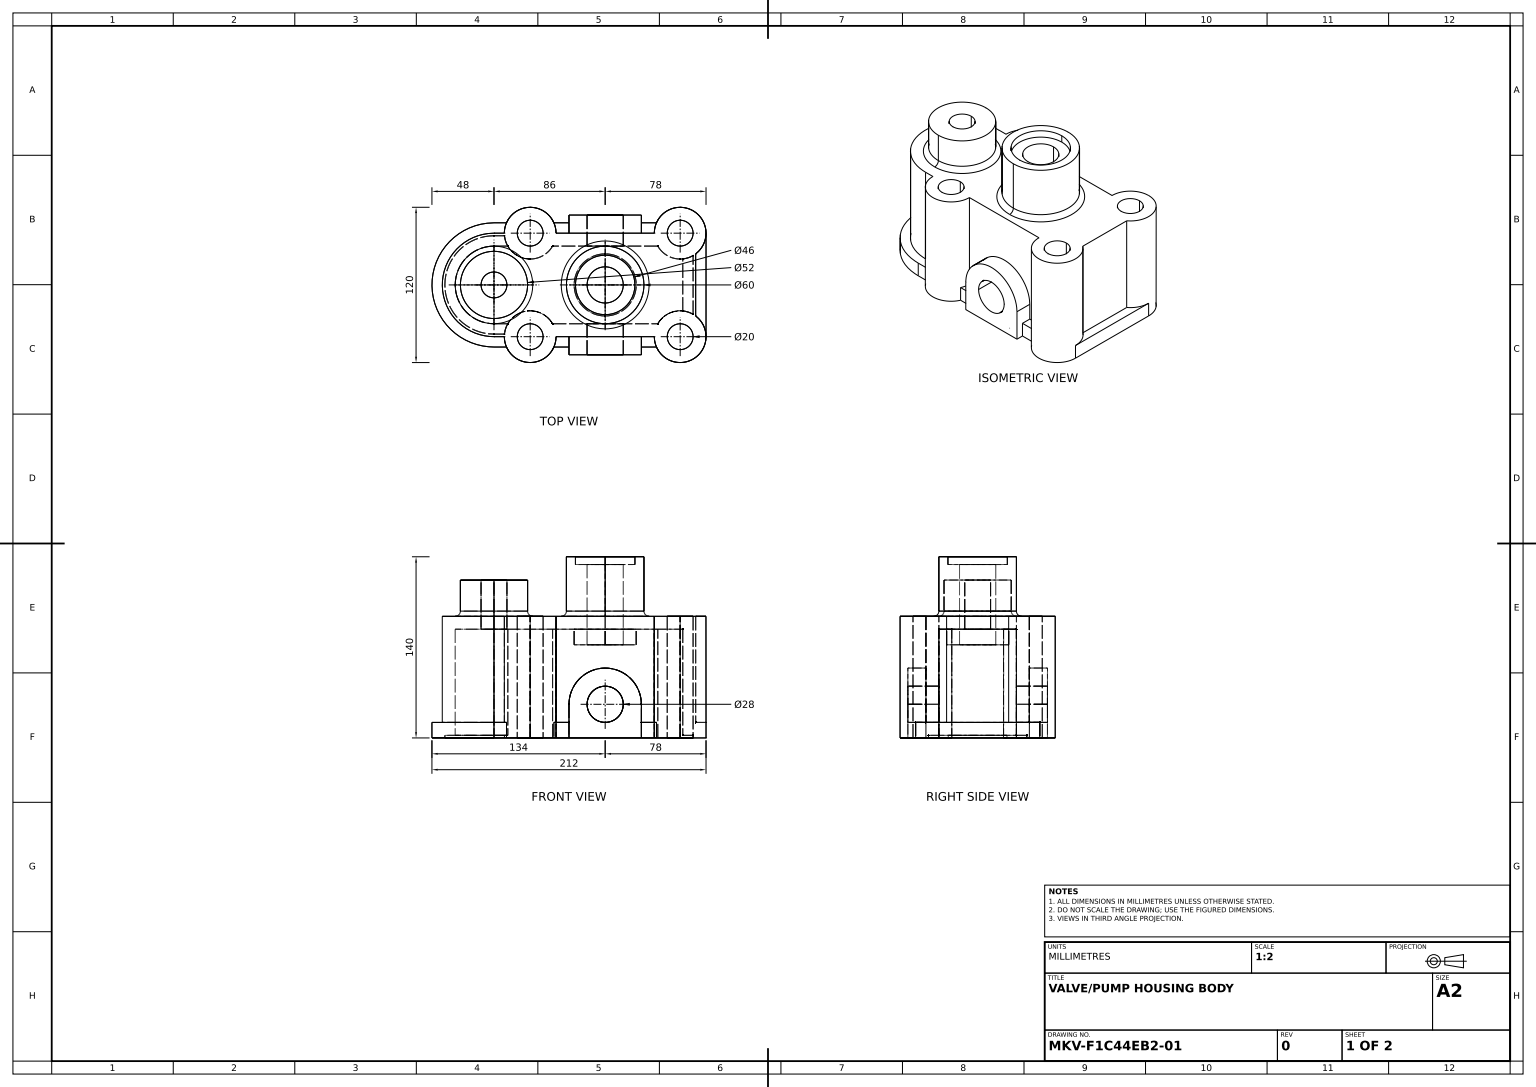
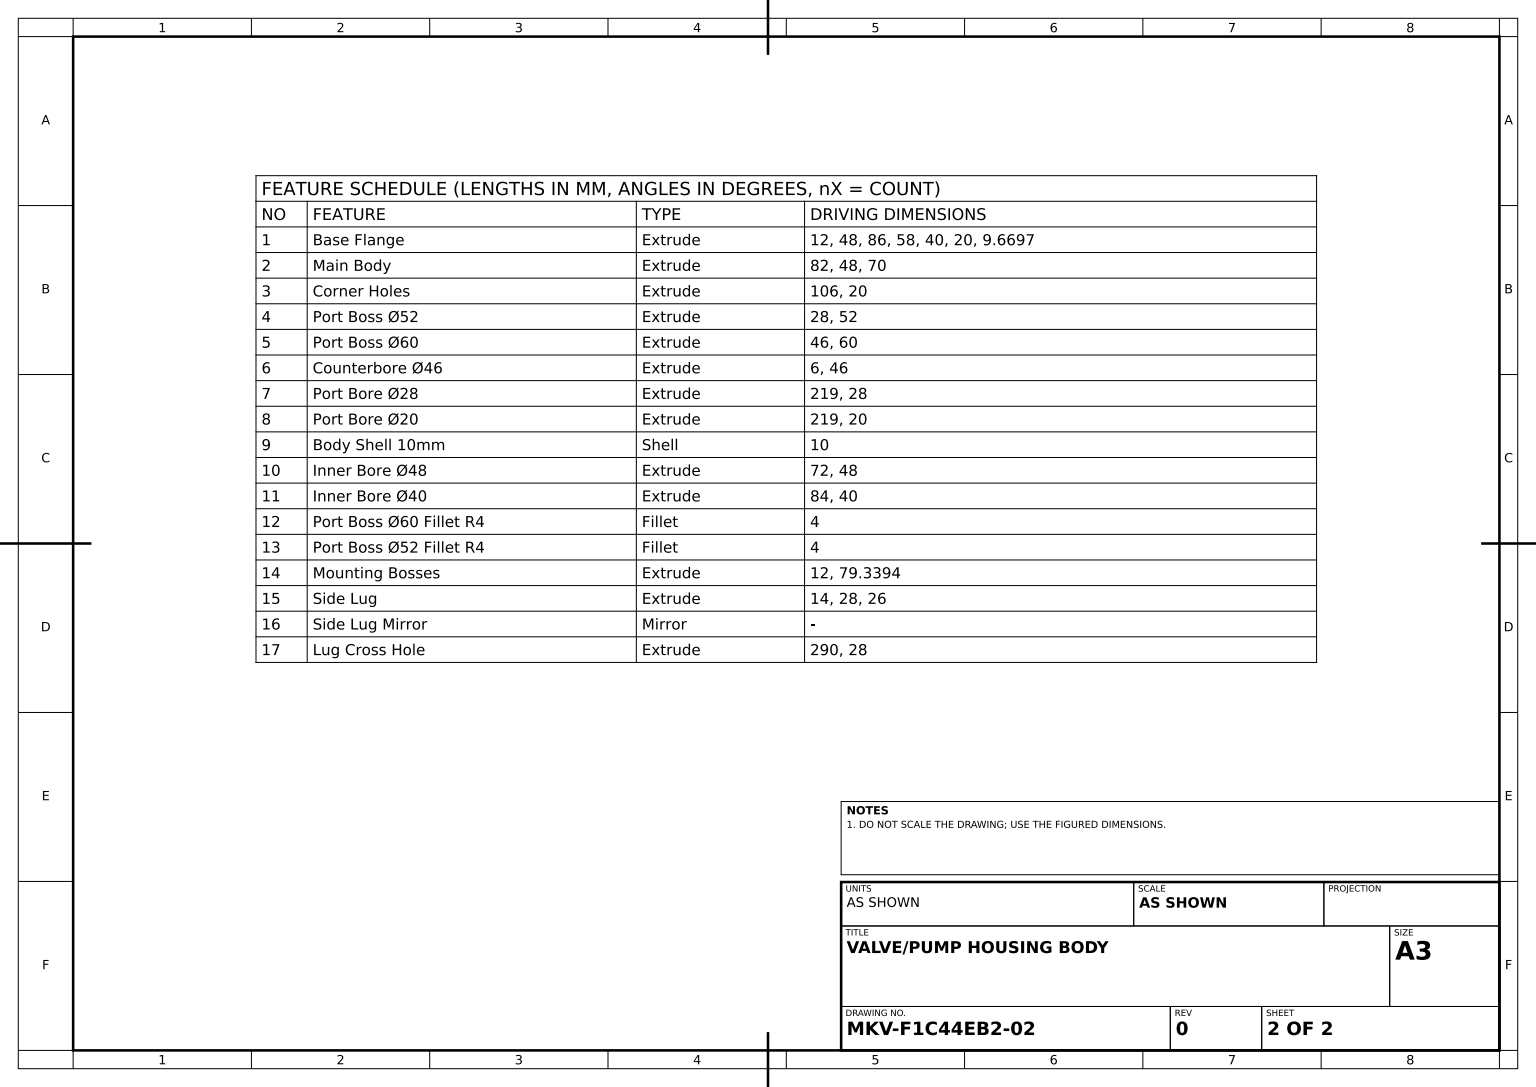
solid
v1 (-86,0,-38)
v2 (-86,0,38)
e1 v1 v2 CIRCLE(AX(P(-86,0,0),D(0,1,0),D(0,0,1)),38)
v3 (-86,2,-38)
e2 v3 v1 LINE
v4 (-86,2,38)
e3 v3 v4 CIRCLE(AX(P(-86,2,0),D(0,1,0),D(0,0,1)),38)
e4 v4 v2 LINE
face CYL(AX(P(-86,12,0),D(0,-1,0),D(0,0,-1)),38) rev [-e1 -e2 e3 e4]
v5 (-77.899749,2,38)
e5 v4 v5 LINE
v6 (-77.899749,0,38)
e6 v6 v5 LINE
e7 v2 v6 LINE
face PLANE(AX(P(-86,12,38),D(0,0,-1),D(-1,0,0))) [-e4 e5 -e6 -e7]
v7 (70,12,24)
v8 (70,12,-24)
e8 v7 v8 LINE
v9 (70,94,-24)
e9 v9 v8 LINE
v10 (70,94,24)
e10 v10 v9 LINE
e11 v10 v7 LINE
face PLANE(AX(P(70,94,0),D(-1,0,0),D(0,0,1))) rev [e8 -e9 -e10 e11]
v11 (-14,26,30)
v12 (-14,26,54)
e12 v11 v12 LINE
v13 (14,26,30)
e13 v11 v13 CIRCLE(AX(P(0,26,30),D(0,0,-1),D(-1,0,0)),14)
v14 (14,26,54)
e14 v13 v14 LINE
e15 v14 v12 CIRCLE(AX(P(0,26,54),D(0,0,1),D(1,0,0)),14)
face CYL(AX(P(0,26,-236),D(0,0,1),D(1,0,0)),14) rev [-e12 e13 e14 e15]
v15 (58,84,-20)
v16 (60,84,-20.100251)
e16 v15 v16 CIRCLE(AX(P(58,84,-40),D(0,1,0),D(0,0,1)),20)
v17 (60,84,20.100251)
e17 v17 v16 LINE
v18 (40.679492,84,30)
e18 v17 v18 CIRCLE(AX(P(58,84,40),D(0,1,0),D(0,0,1)),20)
v19 (-40.679492,84,30)
e19 v19 v18 LINE
v20 (-75.320508,84,30)
e20 v19 v20 CIRCLE(AX(P(-58,84,40),D(0,1,0),D(0,0,1)),20)
v21 (-86,84,30)
e21 v21 v20 LINE
v22 (-86,84,-30)
e22 v22 v21 CIRCLE(AX(P(-86,84,0),D(0,1,0),D(0,0,1)),30)
v23 (-75.320508,84,-30)
e23 v23 v22 LINE
v24 (-58,84,-20)
e24 v23 v24 CIRCLE(AX(P(-58,84,-40),D(0,1,0),D(0,0,1)),20)
v25 (-40.679492,84,-30)
e25 v24 v25 CIRCLE(AX(P(-58,84,-40),D(0,1,0),D(0,0,1)),20)
v26 (40.679492,84,-30)
e26 v26 v25 LINE
e27 v26 v15 CIRCLE(AX(P(58,84,-40),D(0,1,0),D(0,0,1)),20)
v27 (0,84,24)
v28 (0,84,-24)
e28 v27 v28 CIRCLE(AX(P(0,84,0),D(0,1,0),D(0,0,1)),24)
e29 v28 v27 CIRCLE(AX(P(0,84,0),D(0,1,0),D(0,0,1)),24)
v29 (-86,84,-10)
v30 (-86,84,10)
e30 v29 v30 CIRCLE(AX(P(-86,84,0),D(0,1,0),D(0,0,-1)),10)
e31 v30 v29 CIRCLE(AX(P(-86,84,0),D(0,1,0),D(0,0,-1)),10)
face PLANE(AX(P(-86,84,0),D(0,1,0),D(0,0,1))) rev [e16 -e17 e18 -e19 e20 -e21 -e22 -e23 e24 e25 -e26 e27] [e28 e29] [e30 e31]
v31 (-58,94,-50)
v32 (-58,94,-30)
e32 v31 v32 CIRCLE(AX(P(-58,94,-40),D(0,1,0),D(0,0,1)),10)
v33 (-58,0,-30)
e33 v33 v32 LINE
v34 (-58,0,-50)
e34 v34 v33 CIRCLE(AX(P(-58,0,-40),D(0,1,0),D(0,0,1)),10)
e35 v34 v31 LINE
face CYL(AX(P(-58,-12,-40),D(0,1,0),D(0,0,1)),10) rev [e32 -e33 -e34 e35]
v35 (0,72,24)
e36 v35 v27 LINE
v36 (0,72,-24)
e37 v36 v35 CIRCLE(AX(P(0,72,0),D(0,-1,0),D(0,0,-1)),24)
e38 v36 v28 LINE
face CYL(AX(P(0,-85,0),D(0,1,0),D(0,0,1)),24) [-e36 -e37 e38 -e28]
v37 (0,134,23)
v38 (0,140,23)
e39 v37 v38 LINE
v39 (0,140,-23)
e40 v38 v39 CIRCLE(AX(P(0,140,0),D(0,1,0),D(0,0,1)),23)
v40 (0,134,-23)
e41 v40 v39 LINE
e42 v37 v40 CIRCLE(AX(P(0,134,0),D(0,1,0),D(0,0,1)),23)
face CYL(AX(P(0,134,0),D(0,1,0),D(0,0,1)),23) rev [e39 e40 -e41 -e42]
v41 (-39.669697,0,-48)
v42 (-58,0,-60)
e43 v41 v42 CIRCLE(AX(P(-58,0,-40),D(0,1,0),D(0,0,1)),20)
v43 (-58,94,-60)
e44 v43 v42 LINE
v44 (-38,94,-40)
e45 v44 v43 CIRCLE(AX(P(-58,94,-40),D(0,1,0),D(0,0,1)),20)
v45 (-38,12,-40)
e46 v44 v45 LINE
v46 (-39.669697,12,-48)
e47 v45 v46 CIRCLE(AX(P(-58,12,-40),D(0,1,0),D(0,0,-1)),20)
e48 v46 v41 LINE
face CYL(AX(P(-58,12,-40),D(0,-1,0),D(0,0,-1)),20) [e43 -e44 -e45 e46 e47 e48]
v47 (14,26,-54)
v48 (-14,26,-54)
e49 v47 v48 CIRCLE(AX(P(0,26,-54),D(0,0,-1),D(-1,0,0)),14)
v49 (-14,26,-30)
e50 v48 v49 LINE
v50 (14,26,-30)
e51 v49 v50 CIRCLE(AX(P(0,26,-30),D(0,0,1),D(1,0,0)),14)
e52 v47 v50 LINE
face CYL(AX(P(0,26,-236),D(0,0,1),D(1,0,0)),14) rev [e49 e50 e51 -e52]
v51 (-86,2,-30)
e53 v22 v51 LINE
v52 (-75.320508,2,-30)
e54 v52 v51 LINE
e55 v23 v52 LINE
face PLANE(AX(P(-86,94,-30),D(0,0,1),D(1,0,0))) [e53 -e54 -e55 e23]
v53 (58,94,-50)
v54 (58,94,-30)
e56 v53 v54 CIRCLE(AX(P(58,94,-40),D(0,1,0),D(0,0,1)),10)
v55 (58,0,-30)
e57 v55 v54 LINE
v56 (58,0,-50)
e58 v56 v55 CIRCLE(AX(P(58,0,-40),D(0,1,0),D(0,0,1)),10)
e59 v56 v53 LINE
face CYL(AX(P(58,-12,-40),D(0,1,0),D(0,0,1)),10) rev [e56 -e57 -e58 e59]
v57 (-78,12,-40)
v58 (-86,12,-40)
e60 v57 v58 LINE
v59 (-76.330303,12,-48)
e61 v59 v57 CIRCLE(AX(P(-58,12,-40),D(0,1,0),D(0,0,1)),20)
v60 (-86,12,-48)
e62 v59 v60 LINE
v61 (-86,12,48)
e63 v60 v61 CIRCLE(AX(P(-86,12,0),D(0,1,0),D(0,0,1)),48)
v62 (-76.330303,12,48)
e64 v61 v62 LINE
v63 (-78,12,40)
e65 v63 v62 CIRCLE(AX(P(-58,12,40),D(0,1,0),D(0,0,1)),20)
v64 (-86,12,40)
e66 v64 v63 LINE
e67 v58 v64 CIRCLE(AX(P(-86,12,0),D(0,1,0),D(0,0,1)),40)
face PLANE(AX(P(58,12,-40),D(0,1,0),D(0,0,1))) [-e60 -e61 e62 e63 e64 -e65 -e66 -e67]
v65 (0,72,14)
v66 (0,72,-14)
e68 v65 v66 CIRCLE(AX(P(0,72,0),D(0,1,0),D(0,0,-1)),14)
v67 (0,134,14)
e69 v65 v67 LINE
v68 (0,134,-14)
e70 v67 v68 CIRCLE(AX(P(0,134,0),D(0,1,0),D(0,0,1)),14)
e71 v66 v68 LINE
face CYL(AX(P(0,-85,0),D(0,1,0),D(0,0,1)),14) rev [-e68 e69 e70 -e71]
v69 (-77.899749,0,-38)
e72 v69 v1 LINE
v70 (-77.899749,2,-38)
e73 v69 v70 LINE
e74 v70 v3 LINE
face PLANE(AX(P(-86,12,-38),D(0,0,1),D(1,0,0))) [e2 -e72 e73 e74]
v71 (-86,122,-26)
v72 (-86,98,-26)
e75 v71 v72 LINE
v73 (-86,122,26)
e76 v73 v71 CIRCLE(AX(P(-86,122,0),D(0,1,0),D(0,0,1)),26)
v74 (-86,98,26)
e77 v73 v74 LINE
e78 v74 v72 CIRCLE(AX(P(-86,98,0),D(0,1,0),D(0,0,1)),26)
face CYL(AX(P(-86,122,0),D(0,-1,0),D(0,0,-1)),26) [-e75 -e76 e77 e78]
e79 v35 v36 CIRCLE(AX(P(0,72,0),D(0,-1,0),D(0,0,-1)),24)
face CYL(AX(P(0,-85,0),D(0,1,0),D(0,0,1)),24) [-e38 -e79 e36 -e29]
v75 (-76.330303,0,48)
v76 (-39.669697,0,48)
e80 v75 v76 CIRCLE(AX(P(-58,0,40),D(0,1,0),D(0,0,1)),20)
v77 (-39.669697,12,48)
e81 v77 v76 LINE
v78 (-38,12,40)
e82 v77 v78 CIRCLE(AX(P(-58,12,40),D(0,1,0),D(0,0,-1)),20)
v79 (-38,94,40)
e83 v79 v78 LINE
v80 (-78,94,40)
e84 v80 v79 CIRCLE(AX(P(-58,94,40),D(0,1,0),D(0,0,1)),20)
e85 v80 v63 LINE
e86 v62 v75 LINE
face CYL(AX(P(-58,12,40),D(0,-1,0),D(0,0,-1)),20) [e80 -e81 e82 -e83 -e84 e85 e65 e86]
e87 v39 v38 CIRCLE(AX(P(0,140,0),D(0,1,0),D(0,0,1)),23)
e88 v40 v37 CIRCLE(AX(P(0,134,0),D(0,1,0),D(0,0,1)),23)
face CYL(AX(P(0,134,0),D(0,1,0),D(0,0,1)),23) rev [e41 e87 -e39 -e88]
v81 (-28,0,-48)
e89 v41 v81 LINE
v82 (-28,12,-48)
e90 v46 v82 LINE
e91 v81 v82 LINE
face PLANE(AX(P(-39.669697,12,-48),D(0,0,-1),D(-1,0,0))) [-e89 -e48 e90 -e91]
v83 (28,26,-54)
v84 (28,26,-40)
e92 v83 v84 LINE
v85 (28,12,-40)
e93 v85 v84 LINE
v86 (28,12,-48)
e94 v86 v85 LINE
v87 (28,0,-48)
e95 v86 v87 LINE
v88 (28,0,-54)
e96 v88 v87 LINE
e97 v88 v83 LINE
face PLANE(AX(P(28,26,-54),D(1,0,0),D(0,1,0))) [e92 -e93 -e94 e95 -e96 e97]
v89 (-28,26,-54)
v90 (-28,26,-40)
e98 v89 v90 LINE
v91 (-28,0,-54)
e99 v89 v91 LINE
e100 v91 v81 LINE
v92 (-28,12,-40)
e101 v92 v82 LINE
e102 v90 v92 LINE
face PLANE(AX(P(-28,26,-54),D(-1,0,0),D(0,-1,0))) [-e98 e99 e100 e91 -e101 -e102]
v93 (60,2,20.100251)
e103 v17 v93 LINE
v94 (60,2,-20.100251)
e104 v16 v94 LINE
e105 v93 v94 LINE
face PLANE(AX(P(60,94,0),D(-1,0,0),D(0,0,1))) [-e103 e17 e104 -e105]
v95 (-86,94,-30)
v96 (-86,94,30)
e106 v95 v96 CIRCLE(AX(P(-86,94,0),D(0,-1,0),D(0,0,1)),30)
e107 v72 v95 CIRCLE(AX(P(-86,98,-30),D(1,0,0),D(0,0,-1)),4)
e108 v74 v96 CIRCLE(AX(P(-86,98,30),D(-1,0,0),D(0,0,1)),4)
face TORUS(AX(P(-86,98,0),D(0,1,0),D(0,0,1)),30,4) rev [-e106 -e107 -e78 e108]
v97 (-86,2,30)
e109 v51 v97 CIRCLE(AX(P(-86,2,0),D(0,1,0),D(0,0,1)),30)
e110 v21 v97 LINE
face CYL(AX(P(-86,94,0),D(0,-1,0),D(0,0,-1)),30) rev [-e109 -e53 e22 e110]
v98 (58,0,50)
v99 (58,94,50)
e111 v98 v99 LINE
v100 (58,0,30)
e112 v100 v98 CIRCLE(AX(P(58,0,40),D(0,1,0),D(0,0,1)),10)
v101 (58,94,30)
e113 v100 v101 LINE
e114 v101 v99 CIRCLE(AX(P(58,94,40),D(0,1,0),D(0,0,1)),10)
face CYL(AX(P(58,-12,40),D(0,1,0),D(0,0,1)),10) rev [-e111 -e112 e113 e114]
v102 (38,12,-40)
e115 v102 v85 LINE
v103 (39.669697,12,-48)
e116 v103 v102 CIRCLE(AX(P(58,12,-40),D(0,1,0),D(0,0,-1)),20)
e117 v86 v103 LINE
face PLANE(AX(P(58,12,-40),D(0,-1,0),D(0,0,-1))) rev [-e115 -e116 -e117 e94]
v104 (-28,12,40)
v105 (-28,12,48)
e118 v104 v105 LINE
e119 v78 v104 LINE
e120 v105 v77 LINE
face PLANE(AX(P(-58,12,40),D(0,-1,0),D(0,0,-1))) rev [-e118 -e119 -e82 -e120]
v106 (-86,122,-10)
e121 v29 v106 LINE
v107 (-86,122,10)
e122 v30 v107 LINE
e123 v107 v106 CIRCLE(AX(P(-86,122,0),D(0,1,0),D(0,0,1)),10)
face CYL(AX(P(-86,-97,0),D(0,1,0),D(0,0,1)),10) rev [-e121 -e31 e122 e123]
v108 (-86,94,40)
e124 v108 v64 LINE
e125 v108 v80 LINE
face PLANE(AX(P(-86,94,40),D(0,0,-1),D(-1,0,0))) rev [e124 e66 -e85 -e125]
v109 (-75.320508,2,30)
e126 v97 v109 LINE
e127 v5 v109 CIRCLE(AX(P(-58,2,40),D(0,-1,0),D(0,0,1)),20)
e128 v70 v52 CIRCLE(AX(P(-58,2,-40),D(0,1,0),D(0,0,1)),20)
face PLANE(AX(P(58,2,-40),D(0,1,0),D(0,0,1))) rev [e54 e109 e126 -e127 -e5 -e3 -e74 e128]
v110 (0,98,-30)
v111 (0,98,30)
e129 v110 v111 CIRCLE(AX(P(0,98,0),D(0,1,0),D(0,0,1)),30)
v112 (0,140,30)
e130 v112 v111 LINE
v113 (0,140,-30)
e131 v113 v112 CIRCLE(AX(P(0,140,0),D(0,1,0),D(0,0,1)),30)
e132 v113 v110 LINE
face CYL(AX(P(0,140,0),D(0,-1,0),D(0,0,-1)),30) [e129 -e130 -e131 e132]
e133 v106 v107 CIRCLE(AX(P(-86,122,0),D(0,1,0),D(0,0,1)),10)
face CYL(AX(P(-86,-97,0),D(0,1,0),D(0,0,1)),10) rev [-e122 -e30 e121 e133]
e134 v68 v67 CIRCLE(AX(P(0,134,0),D(0,1,0),D(0,0,1)),14)
face PLANE(AX(P(0,134,0),D(0,1,0),D(0,0,1))) [-e134 -e70] [e42 e88]
v114 (39.669697,0,48)
v115 (28,0,48)
e135 v114 v115 LINE
v116 (39.669697,12,48)
e136 v116 v114 LINE
v117 (28,12,48)
e137 v116 v117 LINE
e138 v117 v115 LINE
face PLANE(AX(P(-39.669697,12,48),D(0,0,1),D(1,0,0))) [-e135 -e136 e137 e138]
v118 (28,12,40)
e139 v117 v118 LINE
v119 (38,12,40)
e140 v119 v116 CIRCLE(AX(P(58,12,40),D(0,1,0),D(0,0,-1)),20)
e141 v118 v119 LINE
face PLANE(AX(P(-58,12,40),D(0,-1,0),D(0,0,-1))) rev [-e139 -e137 -e140 -e141]
e142 v20 v109 LINE
v120 (-40.679492,0,30)
e143 v120 v19 LINE
e144 v120 v6 CIRCLE(AX(P(-58,0,40),D(0,1,0),D(0,0,1)),20)
face CYL(AX(P(-58,-12,40),D(0,1,0),D(0,0,1)),20) [-e142 -e20 -e143 e144 e6 e127]
v121 (-76.330303,0,-48)
e145 v42 v121 CIRCLE(AX(P(-58,0,-40),D(0,1,0),D(0,0,1)),20)
e146 v59 v121 LINE
v122 (-78,94,-40)
e147 v122 v57 LINE
e148 v43 v122 CIRCLE(AX(P(-58,94,-40),D(0,1,0),D(0,0,1)),20)
face CYL(AX(P(-58,12,-40),D(0,-1,0),D(0,0,-1)),20) [e44 e145 -e146 e61 -e147 -e148]
e149 v33 v34 CIRCLE(AX(P(-58,0,-40),D(0,1,0),D(0,0,1)),10)
v123 (40.679492,0,30)
e150 v120 v123 LINE
v124 (68,0,22.679492)
e151 v124 v123 CIRCLE(AX(P(58,0,40),D(0,1,0),D(0,0,1)),20)
v125 (68,0,-22.679492)
e152 v124 v125 LINE
v126 (58,0,-20)
e153 v126 v125 CIRCLE(AX(P(58,0,-40),D(0,1,0),D(0,0,1)),20)
v127 (40.679492,0,-30)
e154 v127 v126 CIRCLE(AX(P(58,0,-40),D(0,1,0),D(0,0,1)),20)
v128 (-40.679492,0,-30)
e155 v127 v128 LINE
v129 (-58,0,-20)
e156 v129 v128 CIRCLE(AX(P(-58,0,-40),D(0,1,0),D(0,0,1)),20)
e157 v69 v129 CIRCLE(AX(P(-58,0,-40),D(0,1,0),D(0,0,1)),20)
e158 v98 v100 CIRCLE(AX(P(58,0,40),D(0,1,0),D(0,0,1)),10)
v130 (-58,0,30)
v131 (-58,0,50)
e159 v130 v131 CIRCLE(AX(P(-58,0,40),D(0,1,0),D(0,0,1)),10)
e160 v131 v130 CIRCLE(AX(P(-58,0,40),D(0,1,0),D(0,0,1)),10)
e161 v55 v56 CIRCLE(AX(P(58,0,-40),D(0,1,0),D(0,0,1)),10)
v132 (-28,0,48)
e162 v132 v76 LINE
v133 (-86,0,48)
e163 v133 v75 LINE
v134 (-86,0,-48)
e164 v134 v133 CIRCLE(AX(P(-86,0,0),D(0,1,0),D(0,0,1)),48)
e165 v121 v134 LINE
e166 v91 v88 LINE
v135 (39.669697,0,-48)
e167 v87 v135 LINE
v136 (58,0,-60)
e168 v136 v135 CIRCLE(AX(P(58,0,-40),D(0,1,0),D(0,0,1)),20)
v137 (78,0,-40)
e169 v137 v136 CIRCLE(AX(P(58,0,-40),D(0,1,0),D(0,0,1)),20)
v138 (78,0,40)
e170 v138 v137 LINE
e171 v114 v138 CIRCLE(AX(P(58,0,40),D(0,1,0),D(0,0,1)),20)
v139 (28,0,54)
e172 v139 v115 LINE
v140 (-28,0,54)
e173 v140 v139 LINE
e174 v140 v132 LINE
face PLANE(AX(P(58,0,-40),D(0,1,0),D(0,0,1))) rev [e34 e149] [-e144 e150 -e151 e152 -e153 -e154 e155 -e156 -e157 e72 e1 e7] [e158 e112] [e159 e160] [e58 e161] [e162 -e80 -e163 -e164 -e165 -e145 -e43 e89 -e100 e166 e96 e167 -e168 -e169 -e170 -e171 e135 -e172 -e173 e174]
v141 (38,94,40)
e175 v79 v141 LINE
v142 (-28,26,40)
e176 v142 v104 LINE
v143 (28,26,40)
e177 v143 v142 CIRCLE(AX(P(0,26,40),D(0,0,1),D(1,0,0)),28)
e178 v118 v143 LINE
e179 v141 v119 LINE
face PLANE(AX(P(-38,12,40),D(0,0,-1),D(-1,0,0))) rev [-e175 e83 e119 -e176 -e177 -e178 e141 -e179]
e180 v61 v133 LINE
e181 v60 v134 LINE
face CYL(AX(P(-86,12,0),D(0,-1,0),D(0,0,-1)),48) [-e180 -e63 e181 e164]
e182 v50 v49 CIRCLE(AX(P(0,26,-30),D(0,0,1),D(1,0,0)),14)
e183 v127 v26 LINE
e184 v128 v25 LINE
face PLANE(AX(P(38,12,-30),D(0,0,1),D(1,0,0))) [-e182 -e51] [e183 e26 -e184 -e155]
e185 v71 v73 CIRCLE(AX(P(-86,122,0),D(0,1,0),D(0,0,1)),26)
e186 v72 v74 CIRCLE(AX(P(-86,98,0),D(0,1,0),D(0,0,1)),26)
face CYL(AX(P(-86,122,0),D(0,-1,0),D(0,0,-1)),26) [-e185 e75 e186 -e77]
e187 v84 v90 CIRCLE(AX(P(0,26,-40),D(0,0,1),D(1,0,0)),28)
e188 v83 v89 CIRCLE(AX(P(0,26,-54),D(0,0,1),D(1,0,0)),28)
face CYL(AX(P(0,26,-54),D(0,0,1),D(1,0,0)),28) [e98 -e187 -e92 e188]
v144 (28,26,54)
e189 v144 v143 LINE
v145 (-28,26,54)
e190 v145 v142 LINE
e191 v144 v145 CIRCLE(AX(P(0,26,54),D(0,0,1),D(1,0,0)),28)
face CYL(AX(P(0,26,54),D(0,0,-1),D(-1,0,0)),28) [e189 e177 -e190 -e191]
e192 v139 v144 LINE
face PLANE(AX(P(28,26,54),D(-1,0,0),D(0,-1,0))) rev [e172 -e138 e139 e178 -e189 -e192]
v146 (-58,94,30)
e193 v130 v146 LINE
v147 (-58,94,50)
e194 v146 v147 CIRCLE(AX(P(-58,94,40),D(0,1,0),D(0,0,1)),10)
e195 v131 v147 LINE
face CYL(AX(P(-58,-12,40),D(0,1,0),D(0,0,1)),10) rev [e193 e194 -e195 -e159]
e196 v103 v135 LINE
face PLANE(AX(P(-39.669697,12,-48),D(0,0,-1),D(-1,0,0))) [-e167 -e95 e117 e196]
e197 v132 v105 LINE
face PLANE(AX(P(-39.669697,12,48),D(0,0,1),D(1,0,0))) [e81 -e162 e197 e120]
face PLANE(AX(P(-86,12,-48),D(0,0,1),D(1,0,0))) rev [e165 -e181 -e62 e146]
e198 v99 v101 CIRCLE(AX(P(58,94,40),D(0,1,0),D(0,0,1)),10)
face CYL(AX(P(58,-12,40),D(0,1,0),D(0,0,1)),10) rev [-e158 e111 e198 -e113]
e199 v92 v45 LINE
v148 (38,94,-40)
e200 v148 v44 LINE
e201 v148 v102 LINE
face PLANE(AX(P(38,12,-40),D(0,0,1),D(1,0,0))) rev [e115 e93 e187 e102 e199 -e46 -e200 e201]
v149 (58,94,-60)
e202 v9 v149 CIRCLE(AX(P(58,94,-40),D(0,1,0),D(0,0,1)),20)
v150 (78,12,-40)
e203 v8 v150 CIRCLE(AX(P(58,12,-40),D(0,1,0),D(0,0,1)),20)
e204 v150 v137 LINE
e205 v149 v136 LINE
face CYL(AX(P(58,12,-40),D(0,-1,0),D(0,0,-1)),20) [-e202 e9 e203 e204 e169 -e205]
v151 (0,94,-34)
e206 v110 v151 CIRCLE(AX(P(0,98,-34),D(1,0,0),D(0,0,-1)),4)
v152 (0,94,34)
e207 v152 v151 CIRCLE(AX(P(0,94,0),D(0,-1,0),D(0,0,1)),34)
e208 v111 v152 CIRCLE(AX(P(0,98,34),D(-1,0,0),D(0,0,1)),4)
face TORUS(AX(P(0,98,0),D(0,1,0),D(0,0,1)),34,4) rev [-e129 e206 -e207 -e208]
e209 v111 v110 CIRCLE(AX(P(0,98,0),D(0,1,0),D(0,0,1)),30)
e210 v112 v113 CIRCLE(AX(P(0,140,0),D(0,1,0),D(0,0,1)),30)
face CYL(AX(P(0,140,0),D(0,-1,0),D(0,0,-1)),30) [e209 -e132 -e210 e130]
e211 v145 v140 LINE
face PLANE(AX(P(-28,26,54),D(1,0,0),D(0,1,0))) rev [e118 -e197 -e174 -e211 e190 e176]
e212 v48 v47 CIRCLE(AX(P(0,26,-54),D(0,0,-1),D(-1,0,0)),14)
face PLANE(AX(P(0,26,-54),D(0,0,-1),D(1,0,0))) [-e188 -e97 -e166 -e99] [-e49 -e212]
v153 (78,12,40)
e213 v153 v138 LINE
e214 v153 v7 CIRCLE(AX(P(58,12,40),D(0,1,0),D(0,0,1)),20)
e215 v141 v10 CIRCLE(AX(P(58,94,40),D(0,1,0),D(0,0,1)),20)
face CYL(AX(P(58,12,40),D(0,-1,0),D(0,0,-1)),20) [e140 e136 e171 -e213 e214 -e11 -e215 e179]
e216 v123 v18 LINE
e217 v13 v11 CIRCLE(AX(P(0,26,30),D(0,0,-1),D(-1,0,0)),14)
face PLANE(AX(P(-38,12,30),D(0,0,-1),D(-1,0,0))) [-e216 -e150 e143 e19] [-e13 -e217]
e218 v66 v65 CIRCLE(AX(P(0,72,0),D(0,1,0),D(0,0,-1)),14)
face PLANE(AX(P(0,72,0),D(0,-1,0),D(0,0,-1))) [e37 e79] [e68 e218]
face CYL(AX(P(0,-85,0),D(0,1,0),D(0,0,1)),14) rev [-e69 -e218 e71 e134]
face PLANE(AX(P(58,12,-40),D(0,-1,0),D(0,0,-1))) rev [-e199 e101 -e90 -e47]
e219 v54 v53 CIRCLE(AX(P(58,94,-40),D(0,1,0),D(0,0,1)),10)
face CYL(AX(P(58,-12,-40),D(0,1,0),D(0,0,1)),10) rev [-e161 e57 e219 -e59]
e220 v151 v152 CIRCLE(AX(P(0,94,0),D(0,-1,0),D(0,0,1)),34)
face TORUS(AX(P(0,98,0),D(0,1,0),D(0,0,1)),34,4) rev [-e209 e208 -e220 -e206]
v154 (68,2,22.679492)
e221 v154 v93 CIRCLE(AX(P(58,2,40),D(0,1,0),D(0,0,1)),20)
e222 v124 v154 LINE
face CYL(AX(P(58,-12,40),D(0,1,0),D(0,0,1)),20) [-e18 e103 -e221 -e222 e151 e216]
e223 v153 v150 LINE
face PLANE(AX(P(58,12,-40),D(0,1,0),D(0,0,1))) [-e8 -e214 e223 -e203]
e224 v129 v24 LINE
face CYL(AX(P(-58,-12,-40),D(0,1,0),D(0,0,1)),20) [e184 -e25 -e224 e156]
v155 (-86,94,-40)
e225 v155 v58 LINE
e226 v122 v155 LINE
face PLANE(AX(P(-86,94,-40),D(0,0,1),D(1,0,0))) rev [-e225 -e226 e147 e60]
e227 v96 v95 CIRCLE(AX(P(-86,94,0),D(0,-1,0),D(0,0,1)),30)
face TORUS(AX(P(-86,98,0),D(0,1,0),D(0,0,1)),30,4) rev [-e186 e107 -e227 -e108]
e228 v32 v31 CIRCLE(AX(P(-58,94,-40),D(0,1,0),D(0,0,1)),10)
face CYL(AX(P(-58,-12,-40),D(0,1,0),D(0,0,1)),10) rev [-e35 -e149 e33 e228]
e229 v155 v108 CIRCLE(AX(P(-86,94,0),D(0,1,0),D(0,0,1)),40)
e230 v149 v148 CIRCLE(AX(P(58,94,-40),D(0,1,0),D(0,0,1)),20)
e231 v147 v146 CIRCLE(AX(P(-58,94,40),D(0,1,0),D(0,0,1)),10)
face PLANE(AX(P(-86,94,0),D(0,1,0),D(0,0,1))) [e226 e229 e125 e84 e175 e215 e10 e202 e230 e200 e45 e148] [e207 e220] [-e198 -e114] [-e32 -e228] [-e194 -e231] [-e56 -e219] [e106 e227]
e232 v126 v15 LINE
face CYL(AX(P(58,-12,-40),D(0,1,0),D(0,0,1)),20) [e232 -e27 -e183 e154]
face PLANE(AX(P(-86,122,0),D(0,1,0),D(0,0,1))) [-e123 -e133] [e76 e185]
v156 (68,2,-22.679492)
e233 v125 v156 LINE
e234 v154 v156 LINE
face PLANE(AX(P(68,12,-40),D(-1,0,0),D(0,0,1))) [-e233 -e152 e222 e234]
face CYL(AX(P(-86,94,0),D(0,-1,0),D(0,0,-1)),40) [-e124 -e229 e225 e67]
face CYL(AX(P(0,26,-236),D(0,0,1),D(1,0,0)),14) rev [e182 -e50 e212 e52]
e235 v12 v14 CIRCLE(AX(P(0,26,54),D(0,0,1),D(1,0,0)),14)
face PLANE(AX(P(0,26,54),D(0,0,1),D(1,0,0))) [-e15 -e235] [e211 e173 e192 e191]
face PLANE(AX(P(-86,94,30),D(0,0,-1),D(-1,0,0))) [e142 -e126 -e110 e21]
face CYL(AX(P(-58,-12,40),D(0,1,0),D(0,0,1)),10) rev [e195 e231 -e193 -e160]
face PLANE(AX(P(78,12,-40),D(-1,0,0),D(0,0,1))) rev [e213 e170 -e204 -e223]
face CYL(AX(P(58,12,-40),D(0,-1,0),D(0,0,-1)),20) [e116 -e201 -e230 e205 e168 -e196]
face PLANE(AX(P(0,140,0),D(0,1,0),D(0,0,1))) [e131 e210] [-e87 -e40]
face CYL(AX(P(-58,-12,-40),D(0,1,0),D(0,0,1)),20) [-e128 -e73 e157 e224 -e24 e55]
face CYL(AX(P(0,26,-236),D(0,0,1),D(1,0,0)),14) rev [e12 e235 -e14 e217]
e236 v156 v94 CIRCLE(AX(P(58,2,-40),D(0,-1,0),D(0,0,1)),20)
face PLANE(AX(P(58,2,-40),D(0,1,0),D(0,0,1))) rev [e105 -e236 -e234 e221]
face CYL(AX(P(58,-12,-40),D(0,1,0),D(0,0,1)),20) [-e104 -e16 -e232 e153 e233 e236]
face PLANE(AX(P(-86,12,48),D(0,0,-1),D(-1,0,0))) rev [e180 e163 -e86 -e64]
